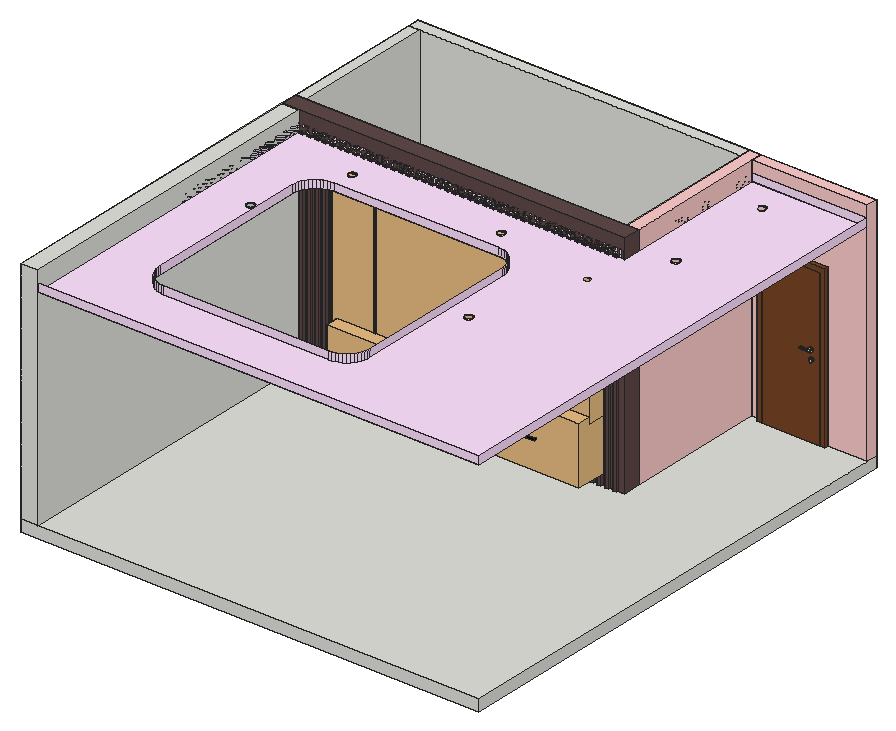
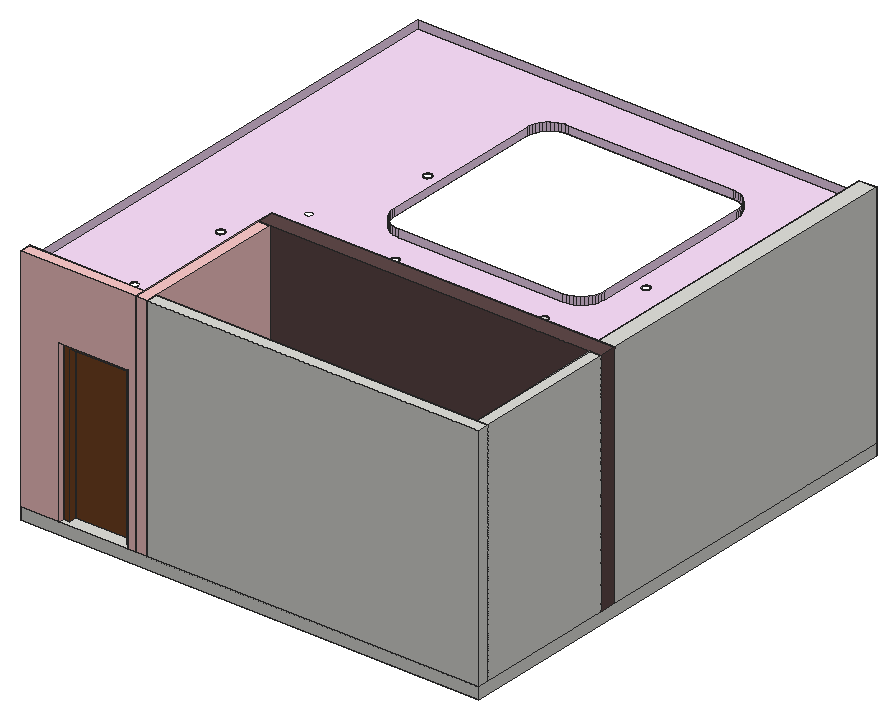
# SketchUp Ruby script. Lengths in inches.
U = 1.inch
M = Sketchup.active_model
def pt(a) = Geom::Point3d.new(a.map { |v| v * U })
def face(e, loops, mat)
  f = e.add_face(loops[0].map { |a| pt(a) })
  loops[1..].each { |l| e.add_face(l.map { |a| pt(a) }).erase! }
  f.material = f.back_material = mat if mat
  f
end
# faces: each face lists its corners as indices into pts; further lists are holes
def faces(e, pts, list, mat = nil) = list.each { |f| face(e, (f[0].is_a?(Array) ? f : [f]).map { |l| l.map { |i| pts[i] } }, mat) }
# xy, xz, yz: faces in a plane at the given z, y or x. An outline is a flat list of corners, or four numbers for a rectangle; further outlines are holes
def ring(l) = l.size == 4 ? [[l[0], l[1]], [l[2], l[1]], [l[2], l[3]], [l[0], l[3]]] : l.each_slice(2).to_a
def flat(e, list, mat, &to3) = list.each { |f| face(e, (f[0].is_a?(Array) ? f : [f]).map { |l| ring(l).map { |u, v| to3.(u, v) } }, mat) }
def xy(e, z, list, mat = nil) = flat(e, list, mat) { |x, y| [x, y, z] }
def xz(e, y, list, mat = nil) = flat(e, list, mat) { |x, z| [x, y, z] }
def yz(e, x, list, mat = nil) = flat(e, list, mat) { |y, z| [x, y, z] }
def lines(e, pts, list) = list.each { |a, b| e.add_line(pt(pts[a]), pt(pts[b])) }
# prism: a flat outline (further loops are holes) pulled along v
def prism(e, loops, v, mat = nil)
  f = face(e, loops, mat); d = Geom::Vector3d.new(v.map { |x| x * U })
  f.pushpull(f.normal.samedirection?(d) ? d.length : -d.length)
end
def box(e, o, s, mat = nil) = prism(e, [[o, [o[0] + s[0], o[1], o[2]], [o[0] + s[0], o[1] + s[1], o[2]], [o[0], o[1] + s[1], o[2]]]], [0, 0, s[2]], mat)
def at(x, y, z, deg = 0) = Geom::Transformation.translation(pt([x, y, z])) * Geom::Transformation.rotation(ORIGIN, Z_AXIS, deg.degrees)
def axes(o, x, y, z) = Geom::Transformation.new([*x, 0, *y, 0, *z, 0, *pt(o).to_a, 1])
def part(name) = M.definitions.add(name)
# library, detail: a bought-in or finely detailed component or shape, given as its bounding box
def library(name, o, s) = part(name).tap { |d| box(d.entities, o, s) }
def detail(e, o, s) = box(e.add_group.entities, o, s)
def put(e, d, t, mat = nil) = e.add_instance(d, t).tap { |i| i.material = mat if mat }
def group(e, t, mat = nil) = e.add_group.tap { |g| g.transformation = t; g.material = mat if mat }.entities
root = M.entities
M.materials.add("[0118_Thistle]").color = [255, 225, 255]
M.materials.add("[0119_RosyBrown]").color = [96, 73, 73]
M.materials.add("[Color A01]").color = [255, 204, 204]
M.materials.add("[Color M00]").color = [255, 255, 255]
M.materials.add("[Color M08]").color = [30, 30, 30]
M.materials.add("[Color M09]").color = [0, 0, 0]
M.materials.add("[Wood Veneer 01]").color = [120, 70, 37]
c1 = part("Group\#4")
box(c1.entities,[0,0,0],[2,1,108])
c2 = library("Group\#11",[0,-15,0],[132.27,15.5,27])
c3 = part("Group\#15")
prism(c3.entities,[[[4.64,1,0],[4.875,1,0],[4.875,0,0],[0,0,0],[0,1,0],[0.23,1,0],[0.23,0.23,0],[4.64,0.23,0]]],[0,0,1.1875])
c4 = library("Group\#13",[0,0,0],[20.18,9.32,59.4])
c5 = library("Group\#7",[0,0,0],[113.2,8.32,59.4])
xy(root,116,[[[9,0,9,171,179.62,171,179.62,254.0625,240,254.0625,240,0],[51.1875,30.1875,137.43,30.1875,139,30.29,140.54,30.6,142.02,31.1,143.43,31.79,144.74,32.67,145.92,33.7,146.95,34.88,147.82,36.1875,148.52,37.59,149.02,39.08,149.33,40.62,149.43,42.1875,149.43,128.8125,149.33,130.38,149.02,131.92,148.52,133.41,147.82,134.8125,146.95,136.12,145.92,137.3,144.74,138.33,143.43,139.21,142.02,139.9,140.54,140.4,139,140.71,137.43,140.8125,51.1875,140.8125,49.62,140.71,48.08,140.4,46.59,139.9,45.1875,139.21,43.88,138.33,42.7,137.3,41.67,136.12,40.79,134.8125,40.1,133.41,39.6,131.92,39.29,130.38,39.1875,128.8125,39.1875,42.1875,39.29,40.62,39.6,39.08,40.1,37.59,40.79,36.1875,41.67,34.88,42.7,33.7,43.88,32.67,45.1875,31.79,46.59,31.1,48.08,30.6,49.62,30.29],[196.98,236.89,197.5,236.95,197.98,237.14,198.4,237.46,198.72,237.87,198.93,238.35,199,238.87,198.94,239.38,198.75,239.87,198.43,240.29,198.02,240.61,197.54,240.8125,197.03,240.89,196.51,240.83,196.02,240.63,195.6,240.32,195.28,239.91,195.08,239.43,195,238.91,195.07,238.39,195.26,237.91,195.57,237.49,195.98,237.17,196.46,236.96],[178.2,146.39,178.72,146.46,179.2,146.66,179.62,146.97,179.9375,147.39,180.14,147.87,180.2,148.39,180.14,148.91,179.9375,149.39,179.62,149.8,179.2,150.12,178.72,150.32,178.2,150.39,177.6875,150.32,177.2,150.12,176.79,149.8,176.47,149.39,176.27,148.91,176.2,148.39,176.27,147.87,176.47,147.39,176.79,146.97,177.2,146.66,177.6875,146.46],[197,180.74,197.52,180.81,198,181,198.42,181.32,198.74,181.74,198.93,182.22,199,182.74,198.93,183.25,198.74,183.74,198.42,184.15,198,184.47,197.52,184.67,197,184.74,196.49,184.67,196,184.47,195.59,184.15,195.27,183.74,195.07,183.25,195,182.74,195.07,182.22,195.27,181.74,195.59,181.32,196,181,196.49,180.81],[48.73,154.34,49.25,154.4,49.73,154.6,50.15,154.92,50.46,155.34,50.66,155.82,50.73,156.34,50.66,156.85,50.46,157.34,50.15,157.75,49.73,158.07,49.25,158.27,48.73,158.34,48.21,158.27,47.73,158.07,47.32,157.75,47,157.34,46.8,156.85,46.73,156.34,46.8,155.82,47,155.34,47.32,154.92,47.73,154.6,48.21,154.4],[126.7,154.34,127.22,154.4,127.7,154.6,128.12,154.92,128.44,155.34,128.64,155.82,128.7,156.34,128.64,156.85,128.44,157.34,128.12,157.75,127.7,158.07,127.22,158.27,126.7,158.34,126.1875,158.27,125.7,158.07,125.29,157.75,124.97,157.34,124.77,156.85,124.7,156.34,124.77,155.82,124.97,155.34,125.29,154.92,125.7,154.6,126.1875,154.4],[160.13,91.36,160.65,91.43,161.13,91.625,161.55,91.94,161.87,92.36,162.07,92.84,162.13,93.36,162.07,93.875,161.87,94.36,161.55,94.77,161.13,95.09,160.65,95.29,160.13,95.36,159.62,95.29,159.13,95.09,158.72,94.77,158.4,94.36,158.2,93.875,158.13,93.36,158.2,92.84,158.4,92.36,158.72,91.94,159.13,91.625,159.62,91.43],[32.11,108.44,32.63,108.51,33.11,108.71,33.53,109.03,33.85,109.44,34.05,109.93,34.11,110.44,34.05,110.96,33.85,111.44,33.53,111.86,33.11,112.18,32.63,112.375,32.11,112.44,31.6,112.375,31.11,112.18,30.7,111.86,30.38,111.44,30.18,110.96,30.11,110.44,30.18,109.93,30.38,109.44,30.7,109.03,31.11,108.71,31.6,108.51]]],"[0118_Thistle]")
xz(root,0,[[9,116,240,120]],"[0118_Thistle]")
xz(root,30.1875,[[51.1875,116,137.43,120]],"[0118_Thistle]")
xz(root,140.8125,[[51.1875,116,137.43,120]],"[0118_Thistle]")
xz(root,171,[[9,116,179.62,120]],"[0118_Thistle]")
xz(root,254.0625,[[179.62,116,240,120]],"[0118_Thistle]")
yz(root,9,[[0,116,171,120]],"[0118_Thistle]")
yz(root,39.1875,[[42.1875,116,128.8125,120]],"[0118_Thistle]")
yz(root,149.43,[[42.1875,116,128.8125,120]],"[0118_Thistle]")
yz(root,179.62,[[171,116,254.0625,120]],"[0118_Thistle]")
yz(root,240,[[0,116,254.0625,120]],"[0118_Thistle]")
p = [[51.1875,30.1875,116],[49.62,30.29,116],[49.62,30.29,120],[51.1875,30.1875,120],[139,30.29,116],[137.43,30.1875,116],
  [137.43,30.1875,120],[139,30.29,120],[48.08,30.6,116],[48.08,30.6,120],[140.54,30.6,116],[140.54,30.6,120],
  [46.59,31.1,116],[46.59,31.1,120],[142.02,31.1,116],[142.02,31.1,120],[45.1875,31.79,116],[45.1875,31.79,120],
  [143.43,31.79,116],[143.43,31.79,120],[43.88,32.67,116],[43.88,32.67,120],[144.74,32.67,116],[144.74,32.67,120],
  [42.7,33.7,116],[42.7,33.7,120],[145.92,33.7,116],[145.92,33.7,120],[41.67,34.88,116],[41.67,34.88,120],
  [146.95,34.88,116],[146.95,34.88,120],[40.79,36.1875,116],[40.79,36.1875,120],[147.82,36.1875,116],[147.82,36.1875,120],
  [40.1,37.59,116],[40.1,37.59,120],[148.52,37.59,116],[148.52,37.59,120],[39.6,39.08,116],[39.6,39.08,120],
  [149.02,39.08,116],[149.02,39.08,120],[39.29,40.62,116],[39.29,40.62,120],[149.33,40.62,116],[149.33,40.62,120],
  [39.1875,42.1875,116],[39.1875,42.1875,120],[149.43,42.1875,116],[149.43,42.1875,120],[159.62,91.43,116],[159.13,91.625,116],
  [159.13,91.625,116.1875],[159.62,91.43,116.1875],[160.13,91.36,116],[160.13,91.36,116.1875],[160.65,91.43,116],[160.65,91.43,116.1875],
  [161.13,91.625,116],[161.13,91.625,116.1875],[158.72,91.94,116],[158.72,91.94,116.1875],[161.55,91.94,116],[161.55,91.94,116.1875],
  [158.4,92.36,116],[158.4,92.36,116.1875],[161.87,92.36,116],[161.87,92.36,116.1875],[158.2,92.84,116],[158.2,92.84,116.1875],
  [162.07,92.84,116],[162.07,92.84,116.1875],[158.13,93.36,116],[158.13,93.36,116.1875],[162.13,93.36,116],[162.13,93.36,116.1875],
  [158.2,93.875,116],[158.2,93.875,116.1875],[162.07,93.875,116],[162.07,93.875,116.1875],[158.4,94.36,116],[158.4,94.36,116.1875],
  [161.87,94.36,116],[161.87,94.36,116.1875],[158.72,94.77,116],[158.72,94.77,116.1875],[161.55,94.77,116],[161.55,94.77,116.1875],
  [159.13,95.09,116],[159.13,95.09,116.1875],[161.13,95.09,116],[161.13,95.09,116.1875],[159.62,95.29,116],[159.62,95.29,116.1875],
  [160.65,95.29,116],[160.65,95.29,116.1875],[160.13,95.36,116],[160.13,95.36,116.1875],[32.11,108.44,116],[31.6,108.51,116],
  [31.6,108.51,116.125],[32.11,108.44,116.125],[32.63,108.51,116],[32.63,108.51,116.125],[31.11,108.71,116],[31.11,108.71,116.125],
  [33.11,108.71,116],[33.11,108.71,116.125],[30.7,109.03,116],[30.7,109.03,116.125],[33.53,109.03,116],[33.53,109.03,116.125],
  [30.38,109.44,116],[30.38,109.44,116.125],[33.85,109.44,116],[33.85,109.44,116.125],[30.18,109.93,116],[30.18,109.93,116.125],
  [34.05,109.93,116],[34.05,109.93,116.125],[30.11,110.44,116],[30.11,110.44,116.125],[34.11,110.44,116],[34.11,110.44,116.125],
  [30.18,110.96,116],[30.18,110.96,116.125],[34.05,110.96,116],[34.05,110.96,116.125],[30.38,111.44,116],[30.38,111.44,116.125],
  [33.85,111.44,116],[33.85,111.44,116.125],[30.7,111.86,116],[30.7,111.86,116.125],[33.53,111.86,116],[33.53,111.86,116.125],
  [31.11,112.18,116],[31.11,112.18,116.125],[33.11,112.18,116],[33.11,112.18,116.125],[31.6,112.375,116],[31.6,112.375,116.125],
  [32.63,112.375,116],[32.63,112.375,116.125],[32.11,112.44,116],[32.11,112.44,116.125],[39.1875,128.8125,116],[39.29,130.38,116],
  [39.29,130.38,120],[39.1875,128.8125,120],[149.33,130.38,116],[149.43,128.8125,116],[149.43,128.8125,120],[149.33,130.38,120],
  [39.6,131.92,116],[39.6,131.92,120],[149.02,131.92,116],[149.02,131.92,120],[40.1,133.41,116],[40.1,133.41,120],
  [148.52,133.41,116],[148.52,133.41,120],[40.79,134.8125,116],[40.79,134.8125,120],[147.82,134.8125,116],[147.82,134.8125,120],
  [41.67,136.12,116],[41.67,136.12,120],[146.95,136.12,116],[146.95,136.12,120],[42.7,137.3,116],[42.7,137.3,120],
  [145.92,137.3,116],[145.92,137.3,120],[43.88,138.33,116],[43.88,138.33,120],[144.74,138.33,116],[144.74,138.33,120],
  [45.1875,139.21,116],[45.1875,139.21,120],[143.43,139.21,116],[143.43,139.21,120],[46.59,139.9,116],[46.59,139.9,120],
  [142.02,139.9,116],[142.02,139.9,120],[48.08,140.4,116],[48.08,140.4,120],[140.54,140.4,116],[140.54,140.4,120],
  [49.62,140.71,116],[49.62,140.71,120],[139,140.71,116],[139,140.71,120],[51.1875,140.8125,116],[51.1875,140.8125,120],
  [137.43,140.8125,116],[137.43,140.8125,120],[48.73,154.34,116],[48.21,154.4,116],[48.21,154.4,116.0625],[48.73,154.34,116.0625],
  [49.25,154.4,116],[49.25,154.4,116.0625],[126.7,154.34,116],[126.1875,154.4,116],[126.1875,154.4,116.125],[126.7,154.34,116.125],
  [127.22,154.4,116],[127.22,154.4,116.125],[47.73,154.6,116],[47.73,154.6,116.0625],[49.73,154.6,116],[49.73,154.6,116.0625],
  [125.7,154.6,116],[125.7,154.6,116.125],[127.7,154.6,116],[127.7,154.6,116.125],[47.32,154.92,116],[47.32,154.92,116.0625],
  [50.15,154.92,116],[50.15,154.92,116.0625],[125.29,154.92,116],[125.29,154.92,116.125],[128.12,154.92,116],[128.12,154.92,116.125],
  [47,155.34,116],[47,155.34,116.0625],[50.46,155.34,116],[50.46,155.34,116.0625],[124.97,155.34,116],[124.97,155.34,116.125],
  [128.44,155.34,116],[128.44,155.34,116.125],[46.8,155.82,116],[46.8,155.82,116.0625],[50.66,155.82,116],[50.66,155.82,116.0625],
  [124.77,155.82,116],[124.77,155.82,116.125],[128.64,155.82,116],[128.64,155.82,116.125],[46.73,156.34,116],[46.73,156.34,116.0625],
  [50.73,156.34,116],[50.73,156.34,116.0625],[124.7,156.34,116],[124.7,156.34,116.125],[128.7,156.34,116],[128.7,156.34,116.125],
  [46.8,156.85,116],[46.8,156.85,116.0625],[50.66,156.85,116],[50.66,156.85,116.0625],[124.77,156.85,116],[124.77,156.85,116.125],
  [128.64,156.85,116],[128.64,156.85,116.125],[47,157.34,116],[47,157.34,116.0625],[50.46,157.34,116],[50.46,157.34,116.0625],
  [124.97,157.34,116],[124.97,157.34,116.125],[128.44,157.34,116],[128.44,157.34,116.125],[47.32,157.75,116],[47.32,157.75,116.0625],
  [50.15,157.75,116],[50.15,157.75,116.0625],[125.29,157.75,116],[125.29,157.75,116.125],[128.12,157.75,116],[128.12,157.75,116.125],
  [47.73,158.07,116],[47.73,158.07,116.0625],[49.73,158.07,116],[49.73,158.07,116.0625],[125.7,158.07,116],[125.7,158.07,116.125],
  [127.7,158.07,116],[127.7,158.07,116.125],[48.21,158.27,116],[48.21,158.27,116.0625],[49.25,158.27,116],[49.25,158.27,116.0625],
  [126.1875,158.27,116],[126.1875,158.27,116.125],[127.22,158.27,116],[127.22,158.27,116.125],[48.73,158.34,116],[48.73,158.34,116.0625],
  [126.7,158.34,116],[126.7,158.34,116.125],[197,180.74,116],[196.49,180.81,116],[196.49,180.81,116.1875],[197,180.74,116.1875],
  [197.52,180.81,116],[197.52,180.81,116.1875],[196,181,116],[196,181,116.1875],[198,181,116],[198,181,116.1875],
  [195.59,181.32,116],[195.59,181.32,116.1875],[198.42,181.32,116],[198.42,181.32,116.1875],[195.27,181.74,116],[195.27,181.74,116.1875],
  [198.74,181.74,116],[198.74,181.74,116.1875],[195.07,182.22,116],[195.07,182.22,116.1875],[198.93,182.22,116],[198.93,182.22,116.1875],
  [195,182.74,116],[195,182.74,116.1875],[199,182.74,116],[199,182.74,116.1875],[195.07,183.25,116],[195.07,183.25,116.1875],
  [198.93,183.25,116],[198.93,183.25,116.1875],[195.27,183.74,116],[195.27,183.74,116.1875],[198.74,183.74,116],[198.74,183.74,116.1875],
  [195.59,184.15,116],[195.59,184.15,116.1875],[198.42,184.15,116],[198.42,184.15,116.1875],[196,184.47,116],[196,184.47,116.1875],
  [198,184.47,116],[198,184.47,116.1875],[196.49,184.67,116],[196.49,184.67,116.1875],[197.52,184.67,116],[197.52,184.67,116.1875],
  [197,184.74,116],[197,184.74,116.1875],[197.98,237.14,116],[197.5,236.95,116],[197.5,236.95,116.1875],[197.98,237.14,116.1875],
  [198.4,237.46,116],[198.4,237.46,116.1875],[198.72,237.87,116],[198.72,237.87,116.1875],[198.93,238.35,116],[198.93,238.35,116.1875],
  [199,238.87,116],[199,238.87,116.1875],[198.94,239.38,116],[198.94,239.38,116.1875],[195.08,239.43,116],[195.28,239.91,116],
  [195.28,239.91,116.1875],[195.08,239.43,116.1875],[198.75,239.87,116],[198.75,239.87,116.1875],[195.6,240.32,116],[195.6,240.32,116.1875],
  [198.43,240.29,116],[198.43,240.29,116.1875],[196.02,240.63,116],[196.02,240.63,116.1875],[198.02,240.61,116],[198.02,240.61,116.1875],
  [196.51,240.83,116],[196.51,240.83,116.1875],[197.54,240.8125,116],[197.54,240.8125,116.1875],[197.03,240.89,116],[197.03,240.89,116.1875],
  [41.37,169.44,42],[55.74,169.44,42],[55.75,161.68,42],[56.75,161.68,42],[57.75,161.68,42],[57.75,169.5,42],
  [57.75,169.68,42],[141.95,169.5,42],[141.95,170,42.24],[141.95,169.68,42.24],[57.75,169.68,42.24],[57.75,161.68,42.24],
  [56.75,161.68,42.24],[55.75,161.68,42.24],[55.62,161.68,42.24],[55.62,162.57,42.24],[55.75,162.57,42.24],[55.75,169.44,42.24],
  [41.42,169.44,42.24],[41.37,170,42.24],[41.15,169.87,42.17],[40.92,169.76,42.1],[40.68,169.66,42.02],[40.44,169.58,41.95],
  [40.2,169.51,41.87],[39.95,169.45,41.79],[39.7,169.41,41.71],[39.44,169.39,41.63],[39.19,169.38,41.55],[38.9375,169.38,41.47],
  [38.68,169.41,41.39],[38.43,169.44,41.31],[38.43,161.68,41.31],[38.43,170,41.31]]
faces(root,p,[[0,1,2,3],[4,5,6,7],[1,8,9,2],[10,4,7,11],[8,12,13,9],[14,10,11,15],[12,16,17,13],[18,14,15,19],
  [16,20,21,17],[22,18,19,23],[20,24,25,21],[26,22,23,27],[24,28,29,25],[30,26,27,31],[28,32,33,29],[34,30,31,35],
  [32,36,37,33],[38,34,35,39],[36,40,41,37],[42,38,39,43],[40,44,45,41],[46,42,43,47],[44,48,49,45],[50,46,47,51],
  [148,149,150,151],[152,153,154,155],[149,156,157,150],[158,152,155,159],[156,160,161,157],[162,158,159,163],[160,164,165,161],[166,162,163,167],
  [164,168,169,165],[170,166,167,171],[168,172,173,169],[174,170,171,175],[172,176,177,173],[178,174,175,179],[176,180,181,177],[182,178,179,183],
  [180,184,185,181],[186,182,183,187],[184,188,189,185],[190,186,187,191],[188,192,193,189],[194,190,191,195],[192,196,197,193],[198,194,195,199]],"[0118_Thistle]")
faces(root,p,[[52,53,54,55],[56,52,55,57],[58,56,57,59],[60,58,59,61],[53,62,63,54],[64,60,61,65],[62,66,67,63],[68,64,65,69],
  [66,70,71,67],[72,68,69,73],[70,74,75,71],[76,72,73,77],[74,78,79,75],[80,76,77,81],[78,82,83,79],[84,80,81,85],
  [82,86,87,83],[88,84,85,89],[86,90,91,87],[92,88,89,93],[90,94,95,91],[96,92,93,97],[94,98,99,95],[98,96,97,99],
  [100,101,102,103],[104,100,103,105],[101,106,107,102],[108,104,105,109],[106,110,111,107],[112,108,109,113],[110,114,115,111],[116,112,113,117],
  [114,118,119,115],[120,116,117,121],[118,122,123,119],[124,120,121,125],[122,126,127,123],[128,124,125,129],[126,130,131,127],[132,128,129,133],
  [130,134,135,131],[136,132,133,137],[134,138,139,135],[140,136,137,141],[138,142,143,139],[144,140,141,145],[142,146,147,143],[146,144,145,147],
  [200,201,202,203],[204,200,203,205],[206,207,208,209],[210,206,209,211],[201,212,213,202],[214,204,205,215],[207,216,217,208],[218,210,211,219],
  [212,220,221,213],[222,214,215,223],[216,224,225,217],[226,218,219,227],[220,228,229,221],[230,222,223,231],[224,232,233,225],[234,226,227,235],
  [228,236,237,229],[238,230,231,239],[232,240,241,233],[242,234,235,243],[236,244,245,237],[246,238,239,247],[240,248,249,241],[250,242,243,251],
  [244,252,253,245],[254,246,247,255],[248,256,257,249],[258,250,251,259],[252,260,261,253],[262,254,255,263],[256,264,265,257],[266,258,259,267],
  [260,268,269,261],[270,262,263,271],[264,272,273,265],[274,266,267,275],[268,276,277,269],[278,270,271,279],[272,280,281,273],[282,274,275,283],
  [276,284,285,277],[286,278,279,287],[280,288,289,281],[290,282,283,291],[284,292,293,285],[292,286,287,293],[288,294,295,289],[294,290,291,295],
  [296,297,298,299],[300,296,299,301],[297,302,303,298],[304,300,301,305],[302,306,307,303],[308,304,305,309],[306,310,311,307],[312,308,309,313],
  [310,314,315,311],[316,312,313,317],[314,318,319,315],[320,316,317,321],[318,322,323,319],[324,320,321,325],[322,326,327,323],[328,324,325,329],
  [326,330,331,327],[332,328,329,333],[330,334,335,331],[336,332,333,337],[334,338,339,335],[340,336,337,341],[338,342,343,339],[342,340,341,343],
  [344,345,346,347],[348,344,347,349],[350,348,349,351],[352,350,351,353],[354,352,353,355],[356,354,355,357],[358,359,360,361],[362,356,357,363],
  [359,364,365,360],[366,362,363,367],[364,368,369,365],[370,366,367,371],[368,372,373,369],[374,370,371,375],[372,376,377,373],[376,374,375,377]],"[Color M00]")
lines(root,p,[[378,379],[380,379],[380,381],[381,382],[382,383],[383,384],[383,385],[386,387],[387,388],[388,389],[389,390],[390,391],
  [391,392],[392,393],[393,394],[394,395],[395,396],[397,398],[398,399],[399,400],[400,401],[401,402],[402,403],[403,404],
  [404,405],[405,406],[406,407],[407,408],[408,409],[410,409],[409,411]])
g1 = group(root,at(0,-60,0))
box(g1,[0,60,0],[240,260.0625,6])
g2 = group(root,at(0,171,6),"[0119_RosyBrown]")
box(g2,[0,0,0],[179.62,9,120])
g3 = group(root,at(0,-60,6))
box(g3,[0,60,0],[9,171,120])
g4 = group(root,at(36.57,164,6),"[0118_Thistle]")
box(g4,[0,0,0],[121.64,6,6])
g5 = group(root,at(10,170,6),"[0119_RosyBrown]")
put(g5,c1,axes([160,0,0],[1,0,0],[0,1,0],[0,0,1.02]))
put(g5,c1,axes([136,0,0],[1,0,0],[0,1,0],[0,0,1.02]))
put(g5,c1,axes([156,0,0],[1,0,0],[0,1,0],[0,0,1.02]))
put(g5,c1,axes([164,0,0],[1,0,0],[0,1,0],[0,0,1.02]))
put(g5,c1,axes([132,0,0],[1,0,0],[0,1,0],[0,0,1.02]))
put(g5,c1,axes([148,0,0],[1,0,0],[0,1,0],[0,0,1.02]))
put(g5,c1,axes([140,0,0],[1,0,0],[0,1,0],[0,0,1.02]))
put(g5,c1,axes([144,0,0],[1,0,0],[0,1,0],[0,0,1.02]))
put(g5,c1,axes([152,0,0],[1,0,0],[0,1,0],[0,0,1.02]))
put(g5,c1,axes([24,0,0],[1,0,0],[0,1,0],[0,0,1.02]))
put(g5,c1,axes([76,0,0],[1,0,0],[0,1,0],[0,0,1.02]))
put(g5,c1,axes([60,0,0],[1,0,0],[0,1,0],[0,0,1.02]))
put(g5,c1,axes([52,0,0],[1,0,0],[0,1,0],[0,0,1.02]))
put(g5,c1,axes([12,0,0],[1,0,0],[0,1,0],[0,0,1.02]))
put(g5,c1,axes([112,0,0],[1,0,0],[0,1,0],[0,0,1.02]))
put(g5,c1,axes([16,0,0],[1,0,0],[0,1,0],[0,0,1.02]))
put(g5,c1,axes([36,0,0],[1,0,0],[0,1,0],[0,0,1.02]))
put(g5,c1,axes([72,0,0],[1,0,0],[0,1,0],[0,0,1.02]))
put(g5,c1,axes([20,0,0],[1,0,0],[0,1,0],[0,0,1.02]))
put(g5,c1,axes([44,0,0],[1,0,0],[0,1,0],[0,0,1.02]))
put(g5,c1,axes([64,0,0],[1,0,0],[0,1,0],[0,0,1.02]))
put(g5,c1,axes([56,0,0],[1,0,0],[0,1,0],[0,0,1.02]))
put(g5,c1,axes([4,0,0],[1,0,0],[0,1,0],[0,0,1.02]))
put(g5,c1,axes([80,0,0],[1,0,0],[0,1,0],[0,0,1.02]))
put(g5,c1,axes([68,0,0],[1,0,0],[0,1,0],[0,0,1.02]))
put(g5,c1,axes([8,0,0],[1,0,0],[0,1,0],[0,0,1.02]))
put(g5,c1,axes([32,0,0],[1,0,0],[0,1,0],[0,0,1.02]))
put(g5,c1,axes([48,0,0],[1,0,0],[0,1,0],[0,0,1.02]))
put(g5,c1,axes([40,0,0],[1,0,0],[0,1,0],[0,0,1.02]))
put(g5,c1,axes([28,0,0],[1,0,0],[0,1,0],[0,0,1.02]))
put(g5,c1,axes([92,0,0],[1,0,0],[0,1,0],[0,0,1.02]))
put(g5,c1,axes([84,0,0],[1,0,0],[0,1,0],[0,0,1.02]))
put(g5,c1,axes([0,0,0],[1,0,0],[0,1,0],[0,0,1.02]))
put(g5,c1,axes([88,0,0],[1,0,0],[0,1,0],[0,0,1.02]))
put(g5,c1,axes([124,0,0],[1,0,0],[0,1,0],[0,0,1.02]))
put(g5,c1,axes([128,0,0],[1,0,0],[0,1,0],[0,0,1.02]))
put(g5,c1,axes([96,0,0],[1,0,0],[0,1,0],[0,0,1.02]))
put(g5,c1,axes([108,0,0],[1,0,0],[0,1,0],[0,0,1.02]))
put(g5,c1,axes([104,0,0],[1,0,0],[0,1,0],[0,0,1.02]))
put(g5,c1,axes([120,0,0],[1,0,0],[0,1,0],[0,0,1.02]))
put(g5,c1,axes([100,0,0],[1,0,0],[0,1,0],[0,0,1.02]))
put(g5,c1,axes([116,0,0],[1,0,0],[0,1,0],[0,0,1.02]))
g6 = group(root,at(173.62,180,6),"[Color A01]")
box(g6,[0,0,0],[6,80.0625,120])
g7 = group(root,at(179.62,254.0625,6),"[Color A01]")
prism(g7,[[[60.38,6,0],[40,6,0],[40,6,84],[4,6,84],[4,6,0],[0,6,0],[0,6,120],[60.38,6,120]]],[0,-6,0])
g8 = group(root,at(183.62,254.0625,6),"[Wood Veneer 01]")
g9 = group(g8,at(0,0,0))
prism(g9,[[[36,3,0],[33,3,0],[33,3,81],[3,3,81],[3,3,0],[0,3,0],[0,3,84],[36,3,84]]],[0,-5,0])
g10 = group(g8,at(3,-2,0))
box(g10,[0,0,0],[30,1,81])
g11 = group(root,at(0,254.0625,6))
box(g11,[0,0,0],[173.62,6,120])
g12 = group(root,at(0,180,6))
box(g12,[0,0,0],[6,74.0625,120])
put(root,c2,axes([36.57,169.5,12],[1,0,0],[0,1,0],[0,0,1.12]),"[Color A01]")
g13 = group(root,at(94.98,156.22,25.66),"[Color M09]")
box(g13,[0,0,0],[15.9375,3.625,2.125])
put(root,c3,at(58.91,153.5,26.71),"[Color M09]")
put(root,c3,at(141.61,153.5,26.71),"[Color M09]")
put(root,c4,axes([33.95,161.67,39],[1.13,0,0],[0,0.89276,0],[0,0,1.1448]),"[Color A01]")
put(root,c5,axes([55.75,161.68,39],[1,0,0],[0,1,0],[0,0,1.1448]),"[Color A01]")
g14 = group(root,at(83.21,162.35,42.24),"[Color M09]")
box(g14,[0,0,0],[38.6875,5.625,4.0625])
g15 = group(root,at(136.22,156.44,42.24),"[0119_RosyBrown]")
box(g15,[-0.625,-1.3125,0],[8.9375,12.125,1.25])
g16 = group(root,at(136.75,158.44,43.49),"[Color M09]")
prism(g16,[[[1.22,5.4375,0],[0,5.4375,0],[0,5.4375,8.25],[0.26,5.4375,9.09],[0.68,5.4375,9.85],[1.24,5.4375,10.48],[1.91,5.4375,10.95],[2.66,5.4375,11.25],[3.45,5.4375,11.35],[4.24,5.4375,11.25],[5,5.4375,10.95],[5.67,5.4375,10.48],[6.23,5.4375,9.85],[6.65,5.4375,9.09],[6.91,5.4375,8.25],[6.91,5.4375,0],[5.69,5.4375,0],[5.69,5.4375,8.02],[5.54,5.4375,8.5],[5.27,5.4375,9],[4.9,5.4375,9.41],[4.46,5.4375,9.72],[3.97,5.4375,9.91],[3.45,5.4375,9.98],[2.9375,5.4375,9.91],[2.45,5.4375,9.72],[2.01,5.4375,9.41],[1.64,5.4375,9],[1.36,5.4375,8.5],[1.22,5.4375,8.02]]],[0,-5.4375,0])
p = [[1.22,5.4375,0],[5.69,5.4375,0]]
lines(g16,p,[[0,1]])
g17 = group(root,at(211.65,251.0625,43.99))
prism(g17,[[[1,1,0],[0.74,1,0.03],[0.5,1,0.13],[0.29,1,0.29],[0.13,1,0.5],[0.03,1,0.74],[0,1,1],[0.03,1,1.26],[0.13,1,1.5],[0.29,1,1.71],[0.5,1,1.87],[0.74,1,1.97],[1,1,2],[1.26,1,1.97],[1.5,1,1.87],[1.71,1,1.71],[1.87,1,1.5],[1.97,1,1.26],[2,1,1],[1.97,1,0.74],[1.87,1,0.5],[1.71,1,0.29],[1.5,1,0.13],[1.26,1,0.03]]],[0,-1,0])
g18 = group(root,at(207.46,250.0625,48.67))
g19 = group(g18,at(3.9375,1,0))
prism(g19,[[[1.6,1,0.2],[1.375,1,0.07],[1.12,1,0],[0.86,1,0],[0.61,1,0.07],[0.38,1,0.2],[0.2,1,0.38],[0.07,1,0.61],[0,1,0.86],[0,1,1.12],[0.07,1,1.375],[0.2,1,1.6],[0.38,1,1.78],[0.61,1,1.92],[0.86,1,1.98],[1.12,1,1.98],[1.375,1,1.92],[1.6,1,1.78],[1.78,1,1.6],[1.92,1,1.375],[1.98,1,1.12],[1.98,1,0.86],[1.92,1,0.61],[1.78,1,0.38]]],[0,-1,0])
g20 = group(g18,at(0,0,0.61))
box(g20,[0,0,0],[5.85,1,0.58])
g21 = group(root,at(73.87,167.68,60),"[Color M08]")
box(g21,[0,0,0],[60.08,2,26.35])
